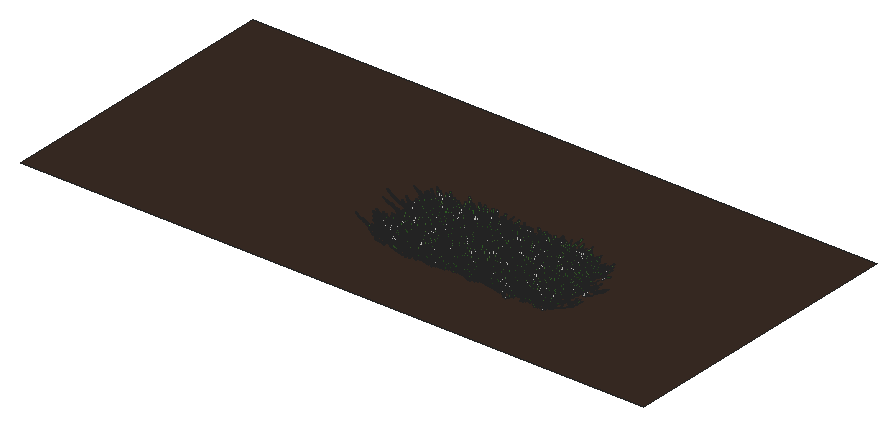
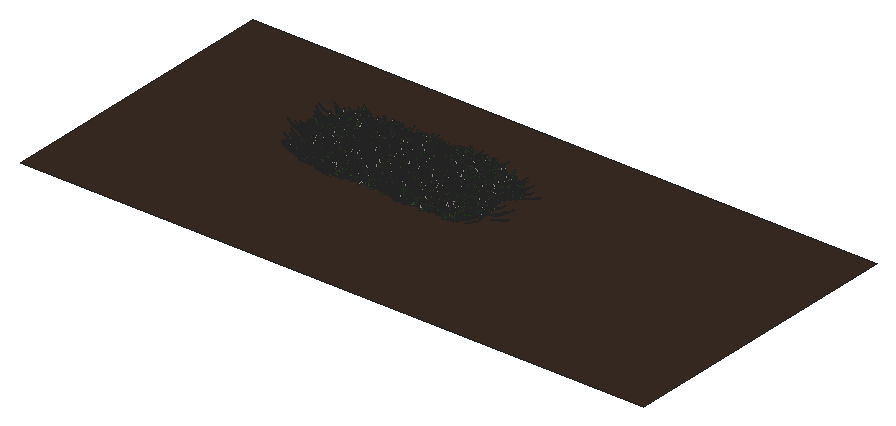
# SketchUp Ruby script. Lengths in inches.
U = 1.inch
M = Sketchup.active_model
def pt(a) = Geom::Point3d.new(a.map { |v| v * U })
def face(e, loops, mat)
  f = e.add_face(loops[0].map { |a| pt(a) })
  loops[1..].each { |l| e.add_face(l.map { |a| pt(a) }).erase! }
  f.material = f.back_material = mat if mat
  f
end
# faces: each face lists its corners as indices into pts; further lists are holes
def faces(e, pts, list, mat = nil) = list.each { |f| face(e, (f[0].is_a?(Array) ? f : [f]).map { |l| l.map { |i| pts[i] } }, mat) }
# xy, xz, yz: faces in a plane at the given z, y or x. An outline is a flat list of corners, or four numbers for a rectangle; further outlines are holes
def ring(l) = l.size == 4 ? [[l[0], l[1]], [l[2], l[1]], [l[2], l[3]], [l[0], l[3]]] : l.each_slice(2).to_a
def flat(e, list, mat, &to3) = list.each { |f| face(e, (f[0].is_a?(Array) ? f : [f]).map { |l| ring(l).map { |u, v| to3.(u, v) } }, mat) }
def xy(e, z, list, mat = nil) = flat(e, list, mat) { |x, y| [x, y, z] }
def xz(e, y, list, mat = nil) = flat(e, list, mat) { |x, z| [x, y, z] }
def yz(e, x, list, mat = nil) = flat(e, list, mat) { |y, z| [x, y, z] }
def lines(e, pts, list) = list.each { |a, b| e.add_line(pt(pts[a]), pt(pts[b])) }
# prism: a flat outline (further loops are holes) pulled along v
def prism(e, loops, v, mat = nil)
  f = face(e, loops, mat); d = Geom::Vector3d.new(v.map { |x| x * U })
  f.pushpull(f.normal.samedirection?(d) ? d.length : -d.length)
end
def box(e, o, s, mat = nil) = prism(e, [[o, [o[0] + s[0], o[1], o[2]], [o[0] + s[0], o[1] + s[1], o[2]], [o[0], o[1] + s[1], o[2]]]], [0, 0, s[2]], mat)
def at(x, y, z, deg = 0) = Geom::Transformation.translation(pt([x, y, z])) * Geom::Transformation.rotation(ORIGIN, Z_AXIS, deg.degrees)
def axes(o, x, y, z) = Geom::Transformation.new([*x, 0, *y, 0, *z, 0, *pt(o).to_a, 1])
def part(name) = M.definitions.add(name)
# library, detail: a bought-in or finely detailed component or shape, given as its bounding box
def library(name, o, s) = part(name).tap { |d| box(d.entities, o, s) }
def detail(e, o, s) = box(e.add_group.entities, o, s)
def put(e, d, t, mat = nil) = e.add_instance(d, t).tap { |i| i.material = mat if mat }
def group(e, t, mat = nil) = e.add_group.tap { |g| g.transformation = t; g.material = mat if mat }.entities
root = M.entities
M.materials.add("Material82").color = [68, 110, 58]
M.materials.add("Material83").color = [48, 90, 38]
M.materials.add("Material84").color = [68, 110, 48]
M.materials.add("Material85").color = [48, 90, 48]
M.materials.add("Material86").color = [58, 110, 58]
M.materials.add("Material87").color = [58, 90, 38]
M.materials.add("Material88").color = [68, 100, 58]
M.materials.add("Material89").color = [48, 100, 38]
M.materials.add("top-soil").color = [58, 44, 36]
c1 = part("grass00")
p = [[-0.6875,0.15,0],[-0.56,0.08,5.52],[-0.04,0.03,2.76],[0.48,-0.02,0],[0.35,-0.02,5.52],[-0.1,-0.14,5.52],
  [-0.12,0.65,8.37],[-0.42,0.65,8.37]]
faces(c1.entities,p,[[0,1,2,3],[3,2,4],[1,5,2],[5,4,2],[1,6,5],[4,5,6],[7,6,1]])
c2 = part("Group16\#1")
put(c2.entities,c1,axes([1.44,-0.61,-0.01],[0.05352,0.12609,0],[-0.10704,0.04543,0.07239],[0.06664,-0.02828,0.11628]),"Material85")
put(c2.entities,c1,axes([0.76,-0.15,-0.01],[0.04676,0.24062,0],[-0.23162,0.04501,0.06642],[0.0652,-0.01267,0.23595]),"Material82")
put(c2.entities,c1,axes([0.79,0.01,-0.01],[-0.00606,0.34651,0],[-0.34381,-0.00602,0.0432],[0.04319,0.00076,0.34386]))
put(c2.entities,c1,axes([1,0.23,-0.01],[-0.07192,0.31144,0],[-0.28722,-0.06632,0.1236],[0.12043,0.02781,0.29478]),"Material84")
put(c2.entities,c1,axes([1.66,0.77,-0.01],[-0.13828,0.29651,0],[-0.21551,-0.1005,0.22471],[0.20365,0.09498,0.23779]),"Material89")
put(c2.entities,c1,axes([0.6875,0.52,-0.01],[-0.18126,0.24051,0],[-0.22746,-0.17142,0.09788],[0.07817,0.05891,0.28481]),"Material84")
put(c2.entities,c1,axes([0.68,0.78,-0.01],[-0.215,0.18688,0],[-0.12385,-0.14248,0.21334],[0.13995,0.16101,0.18878]),"Material82")
put(c2.entities,c1,axes([0.56,1,-0.01],[-0.13756,0.07624,0],[-0.06159,-0.11112,0.0927],[0.04494,0.08108,0.12705]),"Material84")
put(c2.entities,c1,axes([0.2,0.64,-0.01],[-0.23729,0.07254,0],[-0.05711,-0.18681,0.153],[0.04473,0.14632,0.19535]),"Material89")
put(c2.entities,c1,axes([0.0625,0.72,-0.01],[-0.28874,0.02525,0],[-0.02179,-0.24916,0.14647],[0.01276,0.14591,0.25012]),"Material82")
put(c2.entities,c1,axes([-0.08,0.62,-0.01],[-0.34089,-0.04187,0],[0.03255,-0.26504,0.216],[-0.02633,0.21439,0.26703]),"Material89")
put(c2.entities,c1,axes([-0.34,0.98,-0.01],[-0.14314,-0.0493,0],[0.04397,-0.12769,0.06843],[-0.02228,0.0647,0.13505]),"Material89")
put(c2.entities,c1,axes([-0.87,1.45,-0.01],[-0.23488,-0.14114,0],[0.13761,-0.22901,0.06087],[-0.03135,0.05217,0.26717]))
put(c2.entities,c1,axes([-0.72,0.77,-0.01],[-0.14208,-0.13251,0],[0.07209,-0.0773,0.16301],[-0.11118,0.11922,0.1057]),"Material89")
put(c2.entities,c1,axes([-0.62,0.43,-0.01],[-0.14845,-0.21203,0],[0.18654,-0.13061,0.12304],[-0.10079,0.07057,0.22772]),"Material82")
put(c2.entities,c1,axes([-0.68,0.29,-0.01],[-0.13639,-0.32136,0],[0.31723,-0.13464,0.05579],[-0.05136,0.0218,0.34462]),"Material83")
put(c2.entities,c1,axes([-0.64,0.125,-0.01],[-0.0458,-0.23569,0],[0.22124,-0.043,0.08276],[-0.08124,0.01579,0.22538]),"Material86")
put(c2.entities,c1,axes([-1.6,-0.03,-0.01],[0.00576,-0.32897,0],[0.27526,0.00482,0.18018],[-0.18015,-0.00315,0.2753]),"Material84")
put(c2.entities,c1,axes([-1.36,-0.31,-0.01],[0.05718,-0.24765,0],[0.18172,0.04196,0.17267],[-0.16825,-0.03885,0.1865]),"Material89")
put(c2.entities,c1,axes([-1.54,-0.72,-0.01],[0.06537,-0.14017,0],[0.13555,0.06321,0.03939],[-0.0357,-0.01665,0.14956]))
put(c2.entities,c1,axes([-1.19,-0.9,-0.01],[0.09597,-0.12735,0],[0.11214,0.08451,0.07557],[-0.06035,-0.04548,0.14042]),"Material88")
put(c2.entities,c1,axes([-0.47,-0.54,-0.01],[0.11588,-0.10072,0],[0.0618,0.0711,0.12124],[-0.07953,-0.0915,0.0942]))
put(c2.entities,c1,axes([-0.47,-0.84,-0.01],[0.11927,-0.0661,0],[0.06603,0.11913,0.00646],[-0.00313,-0.00565,0.13621]),"Material84")
put(c2.entities,c1,axes([-0.38,-1.24,-0.01],[0.28037,-0.08571,0],[0.0618,0.20215,0.20315],[-0.05939,-0.19428,0.21139]),"Material88")
put(c2.entities,c1,axes([-0.06,-0.66,-0.01],[0.22719,-0.01987,0],[0.01247,0.14255,0.17758],[-0.01547,-0.17691,0.1431]),"Material87")
put(c2.entities,c1,axes([0.11,-0.89,-0.01],[0.14882,0.01828,0],[-0.01058,0.08611,0.12229],[0.01491,-0.12138,0.08676]),"Material85")
put(c2.entities,c1,axes([0.25,-0.72,-0.01],[0.20481,0.07053,0],[-0.06206,0.18022,0.10291],[0.03351,-0.0973,0.1906]),"Material85")
put(c2.entities,c1,axes([0.85,-1.42,-0.01],[0.16481,0.09904,0],[-0.09472,0.15762,0.05616],[0.02893,-0.04814,0.18389]),"Material84")
put(c2.entities,c1,axes([1.01,-1.09,-0.01],[0.21858,0.20385,0],[-0.17495,0.1876,0.15339],[0.10462,-0.11218,0.25652]),"Material89")
put(c2.entities,c1,axes([1.01,-0.71,-0.01],[0.08733,0.12473,0],[-0.06445,0.04512,0.13037],[0.1068,-0.07477,0.07867]),"Material85")
c3 = part("Group15\#1")
put(c3.entities,c2,at(0,0,0))
c4 = part("3darcstudiotree_grass00\#1")
put(c4.entities,c3,at(0,0,0))
xy(root,-34.17,[[596.62,281.03,839.64,394.45]],"top-soil")
put(root,c4,axes([763.98,310.03,-34.17],[-3.54698,0.73807,0],[-1.81276,-1.35492,-0.01893],[-0.04162,-0.0311,1.37131]))
put(root,c4,axes([729.49,310.98,-34.17],[-3.86461,-0.59074,0],[1.45311,-1.4785,-0.05586],[0.12869,-0.13094,1.92103]))
put(root,c4,axes([774.77,311.05,-34.17],[-0.38971,1.40175,0],[-3.70548,-0.16023,-0.02456],[-0.14917,-0.00645,1.70727]))
put(root,c4,axes([738.98,311.33,-34.17],[-3.70591,-0.99796,0],[1.87776,-1.08451,-0.01838],[0.07513,-0.04339,1.80866]))
put(root,c4,axes([763.61,311.37,-34.17],[2.84839,1.04367,0],[-2.27167,0.96426,-0.03885],[-0.20657,0.08768,1.95422]))
put(root,c4,axes([749.69,311.6875,-34.17],[-1.7758,-1.16797,0],[3.11451,-0.73649,-0.04451],[0.21848,-0.05166,1.55797]))
put(root,c4,axes([725.57,311.53,-34.17],[2.01516,1.65729,0],[-3.55056,0.67146,-0.00104],[-0.005,0.00095,1.58037]))
put(root,c4,axes([718.83,312.05,-34.17],[-0.55616,-1.38612,0],[4.6364,-0.28933,-0.05346],[0.22148,-0.01382,1.47567]))
put(root,c4,axes([768.06,312.35,-34.17],[3.94842,-0.68884,0],[1.45256,1.29494,-0.00969],[0.01982,0.01767,1.36001]))
put(root,c4,axes([755.1,312.01,-34.17],[-3.65792,-0.8597,0],[1.995,-1.32021,-0.01663],[0.05672,-0.03754,1.94585]))
put(root,c4,axes([735.8,312.25,-34.17],[-2.06404,-1.37727,0],[3.69374,-0.86095,-0.04139],[0.20463,-0.0477,1.84708]))
put(root,c4,axes([746.11,312.16,-34.17],[-3.29266,-0.34854,0],[0.95777,-1.40726,-0.03217],[0.05606,-0.08237,1.86146]))
put(root,c4,axes([734.125,312.97,-34.17],[3.44047,-0.2055,0],[0.68194,1.77564,-0.05863],[0.04271,0.1112,1.66018]))
put(root,c4,axes([775.31,313.17,-34.17],[3.33641,-0.4539,0],[1.10224,1.26009,-0.03311],[0.06709,0.0767,1.57439]))
put(root,c4,axes([761.11,313.4,-34.17],[4.05026,0.33604,0],[-0.7921,1.48485,-0.04482],[-0.0484,0.09073,1.51278]))
put(root,c4,axes([740.54,312.91,-34.17],[-1.23007,1.60855,0],[-3.72331,-0.44283,-0.01363],[-0.06328,-0.00753,1.41312]))
put(root,c4,axes([757.67,313.31,-34.17],[-4.03093,-0.26709,0],[0.61626,-1.44652,-0.01654],[0.01865,-0.04378,1.89711]))
put(root,c4,axes([744.74,313.83,-34.17],[1.95292,1.06951,0],[-2.86765,0.8144,-0.02117],[-0.10996,0.03123,1.69559]))
put(root,c4,axes([767.63,314.28,-34.17],[4.38423,0.4309,0],[-1.14012,1.80418,-0.03274],[-0.03634,0.0575,1.62193]))
put(root,c4,axes([749.59,314.1,-34.17],[-2.45174,-1.03973,0],[2.50397,-0.91832,-0.03633],[0.18002,-0.06602,1.73438]))
put(root,c4,axes([729.36,314.16,-34.17],[-1.89614,-1.52378,0],[3.69892,-0.71587,-0.01008],[0.04587,-0.00888,1.566]))
put(root,c4,axes([725.65,314.51,-34.17],[3.35774,0.54146,0],[-1.57719,1.52117,-0.03911],[-0.07127,0.06874,1.50402]))
put(root,c4,axes([718,314.1,-34.17],[-3.39635,0.60304,0],[-1.8174,-1.59194,-0.05685],[-0.1325,-0.11606,1.88376]))
put(root,c4,axes([733.41,315.21,-34.17],[3.39282,-0.2362,0],[0.75884,1.6953,-0.03701],[0.03902,0.08718,1.98432]))
put(root,c4,axes([755.73,315.28,-34.17],[0.6087,1.43701,0],[-3.38203,0.22281,-0.00028],[-0.00164,0.00011,1.50491]))
put(root,c4,axes([761.68,316.08,-34.17],[3.17929,-0.7211,0],[2.23361,1.53163,-0.03788],[0.07878,0.05402,1.40078]))
put(root,c4,axes([750.26,315.53,-34.17],[2.01819,1.66422,0],[-3.45385,0.65143,-0.02212],[-0.1358,0.02561,1.95299]))
put(root,c4,axes([744.46,315.7,-34.17],[-0.16089,1.57179,0],[-4.27524,-0.06806,-0.04298],[-0.25282,-0.00402,1.88799]))
put(root,c4,axes([766.61,315.95,-34.17],[-3.05635,-0.6343,0],[1.70161,-1.2752,-0.01604],[0.05188,-0.03888,1.9024]))
put(root,c4,axes([722.87,316.11,-34.17],[0.91536,1.26151,0],[-4.37209,0.4934,-0.02742],[-0.14974,0.0169,1.93645]))
put(root,c4,axes([739.29,316.09,-34.17],[-3.8828,0.51827,0],[-1.09306,-1.27365,-0.02484],[-0.06133,-0.07146,1.96802]))
put(root,c4,axes([728.88,316.45,-34.17],[2.24895,1.38406,0],[-3.92977,0.99312,-0.02786],[-0.13256,0.0335,1.9768]))
put(root,c4,axes([773.76,316.62,-34.17],[-3.21256,-1.12789,0],[2.70503,-1.19832,-0.03256],[0.11538,-0.05111,1.62483]))
put(root,c4,axes([717.24,316.28,-34.17],[-2.03127,1.47153,0],[-3.87167,-0.83121,-0.05406],[-0.22119,-0.04749,1.53936]))
put(root,c4,axes([713.03,316.375,-34.17],[-3.53362,0.69285,0],[-1.78137,-1.413,-0.01143],[-0.02296,-0.01821,1.35283]))
put(root,c4,axes([769.5,317.78,-34.17],[4.62104,-0.01455,0],[0.03483,1.71996,-0.00522],[0.00018,0.00901,1.42947]))
put(root,c4,axes([728.07,317.75,-34.17],[-3.41262,-0.98405,0],[2.00346,-1.0806,-0.03203],[0.14502,-0.07822,1.95145]))
put(root,c4,axes([762.53,318.16,-34.17],[4.2068,0.84458,0],[-2.08885,1.6182,-0.01612],[-0.03432,0.02659,1.61949]))
put(root,c4,axes([724.65,317.9375,-34.17],[-3.8851,-1.03716,0],[2.44189,-1.42264,-0.04034],[0.11257,-0.06558,1.62559]))
put(root,c4,axes([745.24,318.31,-34.17],[4.5376,0.13529,0],[-0.33368,1.74059,-0.04634],[-0.02094,0.10925,1.98901]))
put(root,c4,axes([714.55,318.48,-34.17],[3.81611,-0.29546,0],[0.81359,1.63432,-0.02697],[0.02626,0.05275,1.59996]))
put(root,c4,axes([740.33,318.49,-34.17],[4.2001,-0.13479,0],[0.33266,1.61217,-0.01977],[0.00834,0.04041,1.59866]))
put(root,c4,axes([750.01,318.43,-34.17],[4.12561,0.29265,0],[-0.72369,1.58676,-0.03729],[-0.0346,0.07587,1.60628]))
put(root,c4,axes([775.5625,317.94,-34.17],[-4.01452,0.69277,0],[-1.67449,-1.50916,-0.02625],[-0.04914,-0.04429,1.46233]))
put(root,c4,axes([757.875,318.46,-34.17],[-3.3453,-1.30601,0],[3.28392,-1.30825,-0.03717],[0.14464,-0.05762,1.93537]))
put(root,c4,axes([719.46,318.38,-34.17],[-0.84571,1.33613,0],[-3.59715,-0.35412,-0.00012],[-0.00056,-0.00006,1.39497]))
put(root,c4,axes([736.65,318.8125,-34.17],[1.55645,1.18195,0],[-3.2541,0.66647,-0.04821],[-0.21297,0.04362,1.36797]))
put(root,c4,axes([767.57,319.5,-34.17],[0.41929,-1.46273,0],[4.6699,0.2082,-0.01256],[0.06761,0.00301,1.90836]))
put(root,c4,axes([712.71,319.51,-34.17],[1.28441,1.48375,0],[-3.48852,0.46968,-0.04031],[-0.24472,0.03295,1.77227]))
put(root,c4,axes([758.06,319.89,-34.17],[-1.63649,-1.29377,0],[3.38922,-0.66676,-0.00448],[0.02699,-0.00531,1.90991]))
put(root,c4,axes([752.34,319.75,-34.17],[-2.13819,1.22316,0],[-3.167,-0.86103,-0.02321],[-0.1127,-0.03064,1.70026]))
put(root,c4,axes([727.53,320.25,-34.17],[-2.39621,-0.97294,0],[2.61152,-1.00033,-0.02073],[0.08443,-0.03234,1.5494]))
put(root,c4,axes([762.21,320.59,-34.17],[3.58142,-0.447,0],[1.06233,1.32378,-0.04021],[0.07095,0.08841,1.5432]))
put(root,c4,axes([734.79,320.74,-34.17],[4.64305,-0.03413,0],[0.08366,1.7702,-0.03615],[0.00311,0.0658,1.55355]))
put(root,c4,axes([741.6,320.08,-34.17],[-4.51566,0.3438,0],[-0.75132,-1.53478,-0.00152],[-0.00137,-0.0028,1.41339]))
put(root,c4,axes([723.67,320.93,-34.17],[2.30193,-1.12166,0],[3.41965,1.0915,-0.0352],[0.15447,0.0493,1.86157]))
put(root,c4,axes([744.61,320.59,-34.17],[-3.57945,0.04189,0],[-0.11544,-1.5341,-0.02538],[-0.0045,-0.05977,1.74242]))
put(root,c4,axes([720.06,321.05,-34.17],[3.76479,0.94059,0],[-2.16386,1.34705,-0.03414],[-0.08584,0.05343,1.42377]))
put(root,c4,axes([773.84,320.78,-34.17],[-3.59955,0.15303,0],[-0.4164,-1.52331,-0.01956],[-0.01422,-0.05201,1.97453]))
put(root,c4,axes([729.65,321.72,-34.17],[1.47145,-1.32607,0],[3.01918,0.52105,-0.00213],[0.01031,0.00178,1.30651]))
put(root,c4,axes([734,321.95,-34.17],[2.13019,1.09948,0],[-3.08878,0.93074,-0.0123],[-0.05365,0.01617,1.59876]))
put(root,c4,axes([718.22,321.84,-34.17],[-1.39977,1.36626,0],[-3.55438,-0.56636,-0.02451],[-0.1313,-0.02092,1.66036]))
put(root,c4,axes([762.04,322.68,-34.17],[3.81863,-0.53813,0],[1.40932,1.55539,-0.0155],[0.0332,0.03664,1.9985]))
put(root,c4,axes([740.85,321.92,-34.17],[-3.79382,0.9598,0],[-2.14839,-1.32076,-0.01729],[-0.051,-0.03135,1.62898]))
put(root,c4,axes([772.43,322.59,-34.17],[-3.51388,-0.90483,0],[2.14031,-1.29273,-0.0556],[0.17294,-0.10445,1.66946]))
put(root,c4,axes([722.04,323.23,-34.17],[2.94171,-1.11183,0],[3.18535,1.31078,-0.03986],[0.13301,0.05473,1.66404]))
put(root,c4,axes([746.93,322.85,-34.17],[2.7006,1.1614,0],[-2.43909,0.8821,-0.03804],[-0.19893,0.07194,1.7602]))
put(root,c4,axes([751.52,322.94,-34.17],[-3.12186,-1.16816,0],[2.84193,-1.18123,-0.00166],[0.00643,-0.00267,1.74215]))
put(root,c4,axes([767.625,322.79,-34.17],[-2.88569,0.96312,0],[-2.81786,-1.31311,-0.05904],[-0.17262,-0.08044,1.47981]))
put(root,c4,axes([756.86,322.8,-34.17],[-3.14808,1.22755,0],[-2.57668,-1.02773,-0.03762],[-0.14164,-0.05649,1.47105]))
put(root,c4,axes([733.36,323.95,-34.17],[1.01985,1.24994,0],[-3.27441,0.41552,-0.0339],[-0.22651,0.02874,1.80984]))
put(root,c4,axes([723.4375,324.76,-34.17],[-0.23596,-1.70659,0],[3.32039,-0.0714,-0.01049],[0.06174,-0.00133,1.4693]))
put(root,c4,axes([766.76,324.7,-34.17],[-0.79946,-1.53657,0],[4.27905,-0.34626,-0.03341],[0.18605,-0.01506,1.86102]))
put(root,c4,axes([718.66,324.79,-34.17],[3.51248,0.23364,0],[-0.65189,1.52422,-0.03005],[-0.02625,0.06139,1.54341]))
put(root,c4,axes([762.16,324.54,-34.17],[-3.28059,-1.08182,0],[2.91353,-1.37413,-0.04137],[0.10673,-0.05034,1.36909]))
put(root,c4,axes([740.74,324.66,-34.17],[2.36553,1.18037,0],[-3.06807,0.95629,-0.02315],[-0.10187,0.03175,1.64391]))
put(root,c4,axes([750.69,324.88,-34.17],[2.46344,0.86677,0],[-2.31784,1.02455,-0.00625],[-0.02756,0.01218,1.72796]))
put(root,c4,axes([746.88,324.75,-34.17],[2.29641,1.07421,0],[-2.57105,0.85483,-0.04117],[-0.19383,0.06444,1.55213]))
put(root,c4,axes([729.78,324.66,-34.17],[-2.89048,1.44179,0],[-2.90546,-0.90593,-0.0043],[-0.02277,-0.0071,1.8735]))
put(root,c4,axes([756.69,324.94,-34.17],[0.67214,1.30105,0],[-3.68417,0.29602,-0.04728],[-0.27019,0.02171,1.64346]))
put(root,c4,axes([777.47,325.4,-34.17],[-4.08837,-0.48406,0],[1.24556,-1.63618,-0.01736],[0.02056,-0.027,1.33702]))
put(root,c4,axes([774.77,325.37,-34.17],[-2.8527,1.28628,0],[-3.36111,-1.15935,-0.03347],[-0.14409,-0.0497,1.91416]))
put(root,c4,axes([728.31,326.04,-34.17],[4.59378,0.22046,0],[-0.54654,1.77125,-0.0359],[-0.02405,0.07793,1.88046]))
put(root,c4,axes([769.69,326.41,-34.17],[1.74244,1.18271,0],[-3.27168,0.74965,-0.03711],[-0.19162,0.04391,1.69359]))
put(root,c4,axes([774.98,326.76,-34.17],[-1.03972,-1.40109,0],[4.3795,-0.50546,-0.04795],[0.2061,-0.02379,1.53186]))
put(root,c4,axes([734.33,326.58,-34.17],[-2.79426,-0.70511,0],[1.77672,-1.09506,-0.02395],[0.07288,-0.04492,1.39534]))
put(root,c4,axes([724.34,326.76,-34.17],[-2.68837,-0.8629,0],[2.90522,-1.40773,-0.04334],[0.1065,-0.05161,1.34295]))
put(root,c4,axes([752.95,327.31,-34.17],[2.12809,-1.0558,0],[3.61722,1.13396,-0.06111],[0.24603,0.07713,1.78135]))
put(root,c4,axes([739.01,327.42,-34.17],[0.0983,-1.39772,0],[3.56781,0.03903,-0.00183],[0.01012,0.00011,1.48199]))
put(root,c4,axes([717.43,327.59,-34.17],[4.07348,0.57799,0],[-1.18057,1.29405,-0.01256],[-0.02962,0.03247,1.82155]))
put(root,c4,axes([760.66,327.39,-34.17],[-4.0386,-0.4374,0],[0.94795,-1.36128,-0.02848],[0.0516,-0.0741,1.83531]))
put(root,c4,axes([745.38,327.45,-34.17],[1.35175,1.46561,0],[-4.38115,0.62846,-0.0524],[-0.19286,0.02766,1.36852]))
put(root,c4,axes([755.72,327.56,-34.17],[0.48824,1.58889,0],[-4.56618,0.21822,-0.01569],[-0.06712,0.00321,1.48562]))
put(root,c4,axes([758.95,328.5,-34.17],[3.86781,0.52244,0],[-1.13731,1.30954,-0.02009],[-0.0432,0.04974,1.7458]))
put(root,c4,axes([725.1,328.63,-34.17],[4.03922,-0.03156,0],[0.07296,1.45219,-0.01855],[0.00258,0.0513,1.93628]))
put(root,c4,axes([768.9,328.19,-34.17],[-1.29956,1.24249,0],[-3.63161,-0.59077,-0.01866],[-0.09119,-0.01483,1.55626]))
put(root,c4,axes([736.08,328.29,-34.17],[-4.29389,-0.13256,0],[0.34176,-1.72178,-0.05117],[0.01874,-0.09441,1.54048]))
put(root,c4,axes([762.875,328.66,-34.17],[-2.84597,-0.98358,0],[2.28129,-1.02662,-0.01406],[0.06335,-0.02851,1.77353]))
put(root,c4,axes([718.26,329.28,-34.17],[2.50193,-0.87133,0],[2.32937,1.04026,-0.01409],[0.05813,0.02596,1.64399]))
put(root,c4,axes([741.77,328.99,-34.17],[-4.49069,-0.28234,0],[0.61208,-1.5141,-0.05098],[0.04605,-0.11392,1.67187]))
put(root,c4,axes([730.06,329.6,-34.17],[4.61322,-0.12203,0],[0.30512,1.79396,-0.00473],[0.00139,0.00815,1.49489]))
put(root,c4,axes([745.09,329.34,-34.17],[-2.62594,-1.45094,0],[3.42478,-0.964,-0.01802],[0.06257,-0.01761,1.345]))
put(root,c4,axes([773.33,329,-34.17],[-1.19351,1.65501,0],[-3.6228,-0.40633,-0.01558],[-0.10093,-0.01132,1.90128]))
put(root,c4,axes([749.68,329.74,-34.17],[3.25093,0.54248,0],[-1.41803,1.32165,-0.02719],[-0.07494,0.06985,1.929]))
put(root,c4,axes([713.73,329.53,-34.17],[-3.58514,0.47051,0],[-1.41535,-1.67729,-0.02244],[-0.03437,-0.04073,1.62972]))
put(root,c4,axes([724.2,330.47,-34.17],[4.08766,0.51132,0],[-1.24704,1.55051,-0.00141],[-0.00269,0.00335,1.95289]))
put(root,c4,axes([772.61,330.72,-34.17],[0.81424,-1.34129,0],[3.64589,0.34423,-0.00366],[0.01919,0.00181,1.51551]))
put(root,c4,axes([764.125,330.89,-34.17],[3.6343,-0.40762,0],[1.19135,1.65202,-0.03545],[0.05267,0.07304,1.77295]))
put(root,c4,axes([749.7,330.42,-34.17],[-0.25702,1.50589,0],[-4.4334,-0.11768,-0.01753],[-0.09867,-0.00262,1.87889]))
put(root,c4,axes([769.24,330.55,-34.17],[-3.92506,-0.07313,0],[0.21494,-1.79423,-0.03065],[0.00834,-0.06965,1.9691]))
put(root,c4,axes([742.25,331.07,-34.17],[3.46346,0.58344,0],[-1.61207,1.48838,-0.00364],[-0.00911,0.00841,1.96053]))
put(root,c4,axes([718.15,331.8,-34.17],[1.7154,-1.15643,0],[3.09768,0.71465,-0.02347],[0.14538,0.03354,1.9305]))
put(root,c4,axes([756.04,331.23,-34.17],[-0.11554,1.45354,0],[-4.02615,-0.04978,-0.04067],[-0.20655,-0.00255,1.53414]))
put(root,c4,axes([736.79,331.38,-34.17],[0.845,1.27042,0],[-4.02841,0.41673,-0.05161],[-0.24313,0.02515,1.52021]))
put(root,c4,axes([747.27,331.61,-34.17],[-4.23196,-0.66829,0],[1.43136,-1.40974,-0.04264],[0.09281,-0.09141,1.69007]))
put(root,c4,axes([729.23,331.44,-34.17],[-4.40755,0.3662,0],[-0.80873,-1.51388,-0.00142],[-0.00162,-0.00303,1.63114]))
put(root,c4,axes([713,331.56,-34.17],[-3.77371,1.09403,0],[-2.05317,-1.10148,-0.00523],[-0.01755,-0.00942,1.47184]))
put(root,c4,axes([756.27,332.75,-34.17],[2.10607,-1.53284,0],[3.55653,0.76,-0.00988],[0.05409,0.01156,1.88737]))
put(root,c4,axes([725.54,332.89,-34.17],[1.61408,-1.6002,0],[4.35972,0.68394,-0.04298],[0.19186,0.0301,1.68954]))
put(root,c4,axes([771.99,333.02,-34.17],[-3.98486,0.06108,0],[-0.1339,-1.35868,-0.04521],[-0.01298,-0.1317,1.91035]))
put(root,c4,axes([760.4,333.45,-34.17],[-0.39879,-1.78911,0],[3.98788,-0.13825,-0.04765],[0.27848,-0.00965,1.76037]))
put(root,c4,axes([740.625,333.45,-34.17],[2.70315,0.92974,0],[-3.09727,1.40055,-0.01764],[-0.05733,0.02592,1.74631]))
put(root,c4,axes([753.0625,334.01,-34.17],[3.47556,-0.63984,0],[1.81232,1.53108,-0.02938],[0.06383,0.05392,1.64954]))
put(root,c4,axes([746.29,334.04,-34.17],[2.88826,-0.72218,0],[1.92215,1.1956,-0.03299],[0.1167,0.07259,1.77748]))
put(root,c4,axes([767.87,333.52,-34.17],[-4.37429,0.70017,0],[-1.56113,-1.51689,-0.01879],[-0.03338,-0.03243,1.46955]))
put(root,c4,axes([729.34,333.57,-34.17],[-3.74567,1.07998,0],[-2.52019,-1.35944,-0.03994],[-0.14532,-0.07839,1.97331]))
put(root,c4,axes([719.79,333.84,-34.17],[-1.51727,1.49458,0],[-3.30202,-0.52136,-0.01826],[-0.09361,-0.01478,1.47196]))
put(root,c4,axes([734.93,333.9,-34.17],[-2.53173,1.21264,0],[-2.8931,-0.93942,-0.04557],[-0.23211,-0.07537,1.85346]))
put(root,c4,axes([768.8,335.24,-34.17],[3.99314,-0.58395,0],[1.40862,1.49812,-0.01564],[0.03379,0.03593,1.88746]))
put(root,c4,axes([727.89,335.24,-34.17],[2.23301,-1.20393,0],[2.80312,0.80861,-0.02877],[0.133,0.03837,1.49076]))
put(root,c4,axes([757.92,335.05,-34.17],[3.03872,1.12896,0],[-3.11924,1.30579,-0.01047],[-0.04051,0.01696,1.92288]))
put(root,c4,axes([774.36,335.05,-34.17],[-2.41013,-1.27132,0],[2.91819,-0.86042,-0.02089],[0.0972,-0.02866,1.58683]))
put(root,c4,axes([716.66,334.86,-34.17],[-1.21919,1.74404,0],[-3.47137,-0.37742,-0.03305],[-0.15949,-0.01734,1.35106]))
put(root,c4,axes([738.82,335.3125,-34.17],[4.18586,0.29447,0],[-0.62505,1.38186,-0.04495],[-0.05854,0.12943,1.97854]))
put(root,c4,axes([746.15,335.49,-34.17],[1.93247,1.08024,0],[-2.71059,0.75417,-0.03223],[-0.14585,0.04058,1.37708]))
put(root,c4,axes([733.13,335.86,-34.17],[-2.49297,-0.95003,0],[2.84759,-1.16217,-0.03177],[0.13042,-0.05323,1.8145]))
put(root,c4,axes([724.01,336.1,-34.17],[3.82297,0.44431,0],[-0.93883,1.25636,-0.026],[-0.04711,0.06304,1.59572]))
put(root,c4,axes([760.62,335.94,-34.17],[-3.75498,0.92244,0],[-1.75834,-1.11323,-0.01072],[-0.04199,-0.02659,1.84718]))
put(root,c4,axes([750.18,336.12,-34.17],[0.4621,1.41992,0],[-4.03416,0.20419,-0.0516],[-0.33532,0.01697,1.99718]))
put(root,c4,axes([736.44,337.27,-34.17],[-3.18702,-0.48311,0],[1.45771,-1.49562,-0.04802],[0.08757,-0.08985,1.54794]))
put(root,c4,axes([729.91,337.9,-34.17],[4.11101,0.00408,0],[-0.01055,1.6533,-0.01268],[-0.00019,0.02913,1.83013]))
put(root,c4,axes([750.14,337.57,-34.17],[-2.73846,-0.74739,0],[2.06192,-1.17502,-0.03348],[0.13147,-0.07492,1.87437]))
put(root,c4,axes([764.13,337.86,-34.17],[-2.02199,-1.57321,0],[3.0284,-0.60536,-0.03791],[0.25064,-0.0501,1.88609]))
put(root,c4,axes([773.29,337.55,-34.17],[-3.15684,0.83052,0],[-1.94414,-1.14932,-0.03251],[-0.12313,-0.07279,1.79208]))
put(root,c4,axes([757.87,338.17,-34.17],[2.88281,0.64392,0],[-1.76321,1.22772,-0.02459],[-0.08623,0.06004,1.90817]))
put(root,c4,axes([717.38,337.82,-34.17],[-0.3994,1.69229,0],[-4.36532,-0.16024,-0.02425],[-0.12976,-0.00476,1.76617]))
put(root,c4,axes([740.26,338.35,-34.17],[-0.50603,-1.39331,0],[4.58553,-0.25902,-0.00214],[0.00976,-0.00055,1.59988]))
put(root,c4,axes([724.75,338.22,-34.17],[0.99401,1.39114,0],[-3.81883,0.42439,-0.02067],[-0.11338,0.0126,1.69495]))
put(root,c4,axes([747.55,338.21,-34.17],[0.45996,1.33665,0],[-3.57607,0.19139,-0.02967],[-0.17102,0.00915,1.57371]))
put(root,c4,axes([769.44,338.14,-34.17],[-1.48177,1.26839,0],[-3.97677,-0.72256,-0.00587],[-0.02393,-0.00435,1.47291]))
put(root,c4,axes([733.32,339.12,-34.17],[2.466,-1.02389,0],[3.09141,1.158,-0.03691],[0.15975,0.05984,1.90749]))
put(root,c4,axes([730.9,339.33,-34.17],[3.21693,-1.31198,0],[2.89205,1.10289,-0.03201],[0.144,0.05492,1.88682]))
put(root,c4,axes([757.95,339.26,-34.17],[3.38308,1.28097,0],[-3.13031,1.28579,-0.04664],[-0.1697,0.06971,1.77978]))
put(root,c4,axes([716.9,339.17,-34.17],[-3.15287,0.69435,0],[-1.94177,-1.37131,-0.05669],[-0.17259,-0.12189,1.86391]))
put(root,c4,axes([761.84,339.26,-34.17],[-1.68767,1.14523,0],[-4.10192,-0.94014,-0.02835],[-0.11929,-0.02734,1.73088]))
